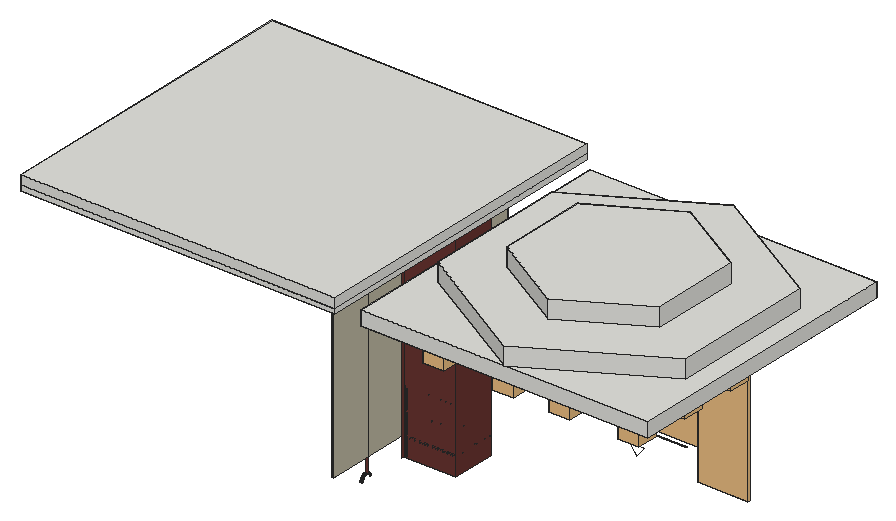
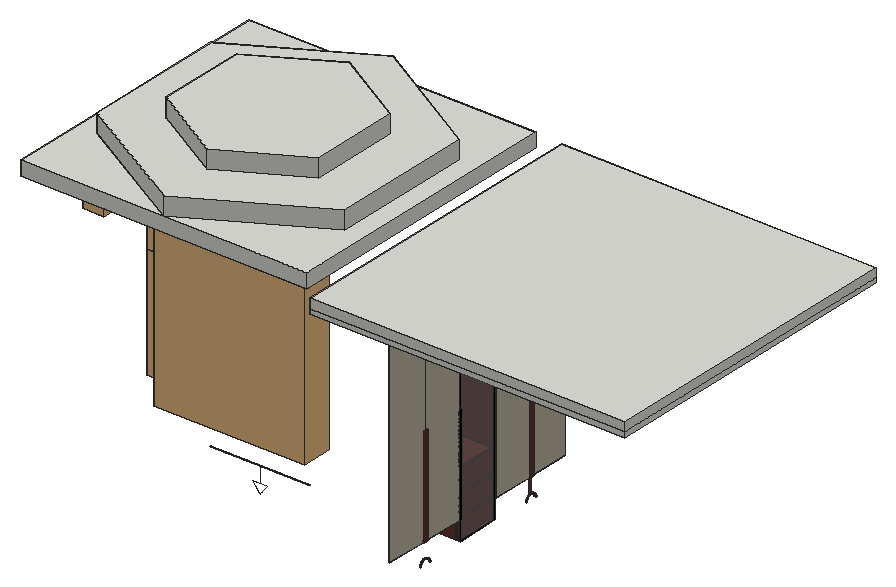
# SketchUp Ruby script. Lengths in millimetres.
U = 1.mm
M = Sketchup.active_model
def pt(a) = Geom::Point3d.new(a.map { |v| v * U })
def face(e, loops, mat)
  f = e.add_face(loops[0].map { |a| pt(a) })
  loops[1..].each { |l| e.add_face(l.map { |a| pt(a) }).erase! }
  f.material = f.back_material = mat if mat
  f
end
# faces: each face lists its corners as indices into pts; further lists are holes
def faces(e, pts, list, mat = nil) = list.each { |f| face(e, (f[0].is_a?(Array) ? f : [f]).map { |l| l.map { |i| pts[i] } }, mat) }
# xy, xz, yz: faces in a plane at the given z, y or x. An outline is a flat list of corners, or four numbers for a rectangle; further outlines are holes
def ring(l) = l.size == 4 ? [[l[0], l[1]], [l[2], l[1]], [l[2], l[3]], [l[0], l[3]]] : l.each_slice(2).to_a
def flat(e, list, mat, &to3) = list.each { |f| face(e, (f[0].is_a?(Array) ? f : [f]).map { |l| ring(l).map { |u, v| to3.(u, v) } }, mat) }
def xy(e, z, list, mat = nil) = flat(e, list, mat) { |x, y| [x, y, z] }
def xz(e, y, list, mat = nil) = flat(e, list, mat) { |x, z| [x, y, z] }
def yz(e, x, list, mat = nil) = flat(e, list, mat) { |y, z| [x, y, z] }
def lines(e, pts, list) = list.each { |a, b| e.add_line(pt(pts[a]), pt(pts[b])) }
# prism: a flat outline (further loops are holes) pulled along v
def prism(e, loops, v, mat = nil)
  f = face(e, loops, mat); d = Geom::Vector3d.new(v.map { |x| x * U })
  f.pushpull(f.normal.samedirection?(d) ? d.length : -d.length)
end
def box(e, o, s, mat = nil) = prism(e, [[o, [o[0] + s[0], o[1], o[2]], [o[0] + s[0], o[1] + s[1], o[2]], [o[0], o[1] + s[1], o[2]]]], [0, 0, s[2]], mat)
def at(x, y, z, deg = 0) = Geom::Transformation.translation(pt([x, y, z])) * Geom::Transformation.rotation(ORIGIN, Z_AXIS, deg.degrees)
def axes(o, x, y, z) = Geom::Transformation.new([*x, 0, *y, 0, *z, 0, *pt(o).to_a, 1])
def part(name) = M.definitions.add(name)
# library, detail: a bought-in or finely detailed component or shape, given as its bounding box
def library(name, o, s) = part(name).tap { |d| box(d.entities, o, s) }
def detail(e, o, s) = box(e.add_group.entities, o, s)
def put(e, d, t, mat = nil) = e.add_instance(d, t).tap { |i| i.material = mat if mat }
def group(e, t, mat = nil) = e.add_group.tap { |g| g.transformation = t; g.material = mat if mat }.entities
root = M.entities
M.materials.add("Olon-Fresh-Linen-VT10-1K").color = [226, 220, 209]
M.materials.add("Tafisa-Chateau-de-Sable-or-Sand-Castle-PM782-2K").color = [163, 138, 119]
M.materials.add("Uniboard-L17-Ambrette-4K").color = [104, 52, 49]
M.materials.add("Uniboard-L19-Putty-4K").color = [187, 181, 160]
M.materials.add("[Color M09]").color = [0, 0, 0]
M.materials.add("[Color M09]1").color = [0, 0, 0]
M.materials.add("[Translucent Glass Gray]").color = [128, 128, 128]
M.materials["[Translucent Glass Gray]"].alpha = 0.5
c1 = part("Group\#6")
prism(c1.entities,[[[0,248.3,178.4],[0,254.5,178.9],[0,259.6,180.5],[0,263.5,183.1],[0,266.3,186.7],[0,268,191.4],[0,268.6,197.1],[0,461,197.1],[0,461,0],[0,0,0],[0,0,197.1],[0,192.4,197.1],[0,193,191.4],[0,194.7,186.7],[0,197.5,183.1],[0,201.4,180.5],[0,206.5,178.9],[0,212.7,178.4]]],[18,0,0])
c2 = part("Group292\#1")
p = [[0,0,0],[0,0,-167.5],[-81.9,0,-167.5],[533.4,-9,0],[-533.4,-9,0],[533.4,9,0],
  [533.4,0,0],[-533.4,9,0],[81.9,0,-167.5],[-533.4,0,0],[0,0,-271.2]]
lines(c2.entities,p,[[0,1],[1,2],[3,4],[5,6],[7,5],[1,8],[9,0],[0,6],[8,10],[4,9],[6,3],[2,10],
  [9,7]])
c3 = part("Rectangle Light\#3")
put(c3.entities,c2,at(0,0,0))
c4 = part("Group\#4")
box(c4.entities,[12,0,-18],[547,461,18])
c5 = part("Group\#7")
prism(c5.entities,[[[20,25.4,1066.8],[20,17.4,1066.8],[20,12.1,1066.3],[20,7.7,1064.9],[20,4.3,1062.5],[20,1.9,1059.1],[20,0.5,1054.7],[20,0,1049.4],[20,0,17.4],[20,0.5,12.1],[20,1.9,7.7],[20,4.3,4.3],[20,7.7,1.9],[20,12.1,0.5],[20,17.4,0],[20,25.4,0]]],[-14,0,0])
c6 = library("Group\#29",[0,0,0],[533.4,18,1202.1])
c7 = library("Group\#23",[0,25.4,-404.8],[1600.2,330.2,1773.4])
c8 = library("Group\#28",[0,0,0],[533.4,18,709.7])
c9 = library("Group\#31",[0,0,0],[226.1,226.1,320.6])
c10 = part("Group\#17")
detail(c10.entities,[87.8,87.8,314.6],[50.5,50.5,6])
g1 = group(c10.entities,at(94.1,94.1,317.8))
xy(g1,0,[[17.2,0,12.4,1.1,8,3.4,4.3,6.8,1.7,11,0.2,15.7,0,20.7,1.1,25.6,3.4,30,6.8,33.6,11,36.3,15.7,37.8,20.7,37.9,25.6,36.8,30,34.5,33.6,31.2,36.3,27,37.8,22.2,37.9,17.2,36.8,12.4,34.5,8,31.2,4.3,27,1.7,22.2,0.2]])
box(root,[2628.9,2293.6,708.2],[18,454.2,2133.6],"Uniboard-L19-Putty-4K")
box(root,[2628.9,879.2,708.2],[18,454.2,2133.6],"Uniboard-L19-Putty-4K")
box(root,[2628.9,1336.4,708.2],[18,454.2,2133.6],"Uniboard-L19-Putty-4K")
xy(root,499.1,[[2628.9,1811.6,2646.9,2272.6]],"[Color M09]")
xy(root,546.1,[[2628.9,1332.9,2631.9,1333.4],[2631.9,1332.9,2646.9,1333.4]],"Tafisa-Chateau-de-Sable-or-Sand-Castle-PM782-2K")
xy(root,546.1,[[2619.9,1332.9,2628.9,1333.4],[2619.9,1336.4,2628.9,1336.9],[2616.9,2747.3,2628.9,2747.8],[2616.9,2750.8,2628.9,2751.3]],"Uniboard-L17-Ambrette-4K")
xy(root,705.2,[[2628.9,2293.6,2646.9,2747.8]],"Tafisa-Chateau-de-Sable-or-Sand-Castle-PM782-2K")
xy(root,705.2,[[2628.9,879.2,2646.9,1333.4],[2628.9,1336.4,2646.9,1790.6],[2628.9,2750.8,2646.9,3205]],"Uniboard-L17-Ambrette-4K")
xy(root,708.2,[[2628.9,2750.8,2646.9,3205]],"Uniboard-L19-Putty-4K")
xy(root,2823.8,[[2628.9,1811.6,2646.9,2272.6],[2649.9,1811.6,3208.9,2272.6]],"Uniboard-L17-Ambrette-4K")
xy(root,2841.8,[[2646.9,1793.6,2649.9,2290.6],[2628.9,2750.8,2646.9,3205]],"Uniboard-L19-Putty-4K")
xy(root,2841.8,[[2628.9,1793.6,2646.9,2290.6]],"[Color M09]")
xy(root,2844.8,[[2628.9,879.2,2646.9,3208]],"Uniboard-L19-Putty-4K")
xy(root,2895.6,[[2628.9,879.2,2646.9,3258.8],[2646.9,879.2,3238.5,3258.8]],"Uniboard-L19-Putty-4K")
xy(root,3048,[[5171.3,0,3851.4,762,3851.4,2286,5171.3,3048,6491.1,2286,6491.1,762]])
xy(root,3241.7,[[[5171.3,0,6491.1,762,6491.1,2286,5171.3,3048,3851.4,2286,3851.4,762],[5171.3,580.4,4354.1,1052.2,4354.1,1995.8,5171.3,2467.6,5988.4,1995.8,5988.4,1052.2]]])
xy(root,3435.4,[[5171.3,580.4,5988.4,1052.2,5988.4,1995.8,5171.3,2467.6,4354.1,1995.8,4354.1,1052.2]])
xz(root,879.2,[[2628.9,2844.8,2646.9,2895.6]],"Uniboard-L19-Putty-4K")
xz(root,1333.4,[[2628.9,546.1,2646.9,705.2]],"Uniboard-L17-Ambrette-4K")
xz(root,1811.6,[[2649.9,499.1,3208.9,2823.8]],"Uniboard-L17-Ambrette-4K")
xz(root,1811.6,[[2628.9,499.1,2646.9,2823.8]],"[Color M09]")
xz(root,2272.6,[[2649.9,499.1,3208.9,2823.8]],"Uniboard-L17-Ambrette-4K")
xz(root,2272.6,[[2628.9,499.1,2646.9,2823.8]],"[Color M09]")
xz(root,2750.8,[[2628.9,708.2,2646.9,2841.8]],"Uniboard-L19-Putty-4K")
xz(root,3205,[[2628.9,708.2,2646.9,2841.8]],"Uniboard-L19-Putty-4K")
yz(root,2628.9,[[2750.8,708.2,3205,2841.8]],"Uniboard-L19-Putty-4K")
yz(root,2637.9,[[1811.6,499.1,2272.6,2823.8]],"[Translucent Glass Gray]")
yz(root,2646.9,[[1793.6,499.1,1811.6,2823.8],[1793.6,2823.8,2290.6,2841.8]],"[Color M09]")
yz(root,2649.9,[[1793.6,499.1,1811.6,2823.8],[1793.6,2823.8,2290.6,2841.8]],"Uniboard-L17-Ambrette-4K")
yz(root,3208.9,[[1811.6,499.1,2272.6,2823.8]],"Uniboard-L17-Ambrette-4K")
yz(root,3851.4,[[762,3048,2286,3241.7]])
yz(root,4354.1,[[1052.2,3241.7,1995.8,3435.4]])
yz(root,5988.4,[[1052.2,3241.7,1995.8,3435.4]])
yz(root,6491.1,[[762,3048,2286,3241.7]])
p = [[2646.9,1270.2,487.2],[2631.9,1270.2,487.2],[2631.9,1270.4,489.2],[2646.9,1270.4,489.2],[2628.9,1270.4,489.2],[2628.9,1270.7,491.3],
  [2619.9,1270.7,491.3],[2619.9,1270.4,489.2],[2631.9,1270.7,491.3],[2646.9,1270.7,491.3],[2628.9,1399.1,491.3],[2628.9,1399.4,489.2],
  [2619.9,1399.4,489.2],[2619.9,1399.1,491.3],[2628.9,2684.8,489.2],[2628.9,2685.1,491.3],[2616.9,2685.1,491.3],[2616.9,2684.8,489.2],
  [2628.9,2813.5,491.3],[2628.9,2813.8,489.2],[2616.9,2813.8,489.2],[2616.9,2813.5,491.3],[2628.9,1271.1,493.3],[2619.9,1271.1,493.3],
  [2631.9,1271.1,493.3],[2646.9,1271.1,493.3],[2628.9,1398.8,493.3],[2619.9,1398.8,493.3],[2628.9,2685.5,493.3],[2616.9,2685.5,493.3],
  [2628.9,2813.2,493.3],[2616.9,2813.2,493.3],[2628.9,1271.5,495.3],[2619.9,1271.5,495.3],[2631.9,1271.5,495.3],[2646.9,1271.5,495.3],
  [2628.9,1398.3,495.3],[2619.9,1398.3,495.3],[2628.9,2685.9,495.3],[2616.9,2685.9,495.3],[2628.9,2812.7,495.3],[2616.9,2812.7,495.3],
  [2628.9,1271.9,497.3],[2619.9,1271.9,497.3],[2631.9,1271.9,497.3],[2646.9,1271.9,497.3],[2628.9,1397.9,497.3],[2619.9,1397.9,497.3],
  [2628.9,2686.3,497.3],[2616.9,2686.3,497.3],[2628.9,2812.3,497.3],[2616.9,2812.3,497.3],[2628.9,1272.5,499.2],[2619.9,1272.5,499.2],
  [2631.9,1272.5,499.2],[2646.9,1272.5,499.2],[2628.9,1397.3,499.2],[2619.9,1397.3,499.2],[2628.9,2686.9,499.2],[2616.9,2686.9,499.2],
  [2628.9,2811.7,499.2],[2616.9,2811.7,499.2],[2628.9,1273.1,501.2],[2619.9,1273.1,501.2],[2631.9,1273.1,501.2],[2646.9,1273.1,501.2],
  [2628.9,1396.7,501.2],[2619.9,1396.7,501.2],[2628.9,2687.5,501.2],[2616.9,2687.5,501.2],[2628.9,2811.1,501.2],[2616.9,2811.1,501.2],
  [2628.9,1273.7,503.1],[2619.9,1273.7,503.1],[2631.9,1273.7,503.1],[2646.9,1273.7,503.1],[2628.9,1396.1,503.1],[2619.9,1396.1,503.1],
  [2628.9,2688.1,503.1],[2616.9,2688.1,503.1],[2628.9,2810.5,503.1],[2616.9,2810.5,503.1],[2628.9,1274.5,505],[2619.9,1274.5,505],
  [2631.9,1274.5,505],[2646.9,1274.5,505],[2628.9,1395.3,505],[2619.9,1395.3,505],[2628.9,2688.9,505],[2616.9,2688.9,505],
  [2628.9,2809.7,505],[2616.9,2809.7,505],[2628.9,1275.3,506.9],[2619.9,1275.3,506.9],[2631.9,1275.3,506.9],[2646.9,1275.3,506.9],
  [2628.9,1394.6,506.9],[2619.9,1394.6,506.9],[2628.9,2689.7,506.9],[2616.9,2689.7,506.9],[2628.9,2809,506.9],[2616.9,2809,506.9],
  [2628.9,1276.1,508.8],[2619.9,1276.1,508.8],[2631.9,1276.1,508.8],[2646.9,1276.1,508.8],[2628.9,1393.7,508.8],[2619.9,1393.7,508.8],
  [2628.9,2690.5,508.8],[2616.9,2690.5,508.8],[2628.9,2808.1,508.8],[2616.9,2808.1,508.8],[2628.9,1277,510.6],[2619.9,1277,510.6],
  [2631.9,1277,510.6],[2646.9,1277,510.6],[2628.9,1392.8,510.6],[2619.9,1392.8,510.6],[2628.9,2691.4,510.6],[2616.9,2691.4,510.6],
  [2628.9,2807.2,510.6],[2616.9,2807.2,510.6],[2628.9,1277.9,512.4],[2619.9,1277.9,512.4],[2631.9,1277.9,512.4],[2646.9,1277.9,512.4],
  [2628.9,1391.9,512.4],[2619.9,1391.9,512.4],[2628.9,2692.3,512.4],[2616.9,2692.3,512.4],[2628.9,2806.3,512.4],[2616.9,2806.3,512.4],
  [2628.9,1279,514.2],[2619.9,1279,514.2],[2631.9,1279,514.2],[2646.9,1279,514.2],[2628.9,1390.9,514.2],[2619.9,1390.9,514.2],
  [2628.9,2693.4,514.2],[2616.9,2693.4,514.2],[2628.9,2805.3,514.2],[2616.9,2805.3,514.2],[2628.9,1280,515.9],[2619.9,1280,515.9],
  [2631.9,1280,515.9],[2646.9,1280,515.9],[2628.9,1389.8,515.9],[2619.9,1389.8,515.9],[2628.9,2694.4,515.9],[2616.9,2694.4,515.9],
  [2628.9,2804.2,515.9],[2616.9,2804.2,515.9],[2628.9,1281.1,517.6],[2619.9,1281.1,517.6],[2631.9,1281.1,517.6],[2646.9,1281.1,517.6],
  [2628.9,1388.7,517.6],[2619.9,1388.7,517.6],[2628.9,2695.5,517.6],[2616.9,2695.5,517.6],[2628.9,2803.1,517.6],[2616.9,2803.1,517.6],
  [2628.9,1282.3,519.3],[2619.9,1282.3,519.3],[2631.9,1282.3,519.3],[2646.9,1282.3,519.3],[2628.9,1387.5,519.3],[2619.9,1387.5,519.3],
  [2628.9,2696.7,519.3],[2616.9,2696.7,519.3],[2628.9,2801.9,519.3],[2616.9,2801.9,519.3],[2628.9,1283.5,520.9],[2619.9,1283.5,520.9],
  [2631.9,1283.5,520.9],[2646.9,1283.5,520.9],[2628.9,1386.3,520.9],[2619.9,1386.3,520.9],[2628.9,2697.9,520.9],[2616.9,2697.9,520.9],
  [2628.9,2800.7,520.9],[2616.9,2800.7,520.9],[2628.9,1284.8,522.5],[2619.9,1284.8,522.5],[2631.9,1284.8,522.5],[2646.9,1284.8,522.5],
  [2628.9,1385,522.5],[2619.9,1385,522.5],[2628.9,2699.2,522.5],[2616.9,2699.2,522.5],[2628.9,2799.4,522.5],[2616.9,2799.4,522.5],
  [2628.9,1286.1,524.1],[2619.9,1286.1,524.1],[2631.9,1286.1,524.1],[2646.9,1286.1,524.1],[2628.9,1383.7,524.1],[2619.9,1383.7,524.1],
  [2628.9,2700.5,524.1],[2616.9,2700.5,524.1],[2628.9,2798.1,524.1],[2616.9,2798.1,524.1],[2628.9,1287.5,525.6],[2619.9,1287.5,525.6],
  [2631.9,1287.5,525.6],[2646.9,1287.5,525.6],[2628.9,1382.3,525.6],[2619.9,1382.3,525.6],[2628.9,2701.9,525.6],[2616.9,2701.9,525.6],
  [2628.9,2796.7,525.6],[2616.9,2796.7,525.6],[2628.9,1288.9,527.1],[2619.9,1288.9,527.1],[2631.9,1288.9,527.1],[2646.9,1288.9,527.1],
  [2628.9,1380.9,527.1],[2619.9,1380.9,527.1],[2628.9,2703.3,527.1],[2616.9,2703.3,527.1],[2628.9,2795.3,527.1],[2616.9,2795.3,527.1],
  [2628.9,1290.4,528.5],[2619.9,1290.4,528.5],[2631.9,1290.4,528.5],[2646.9,1290.4,528.5],[2628.9,1379.4,528.5],[2619.9,1379.4,528.5],
  [2628.9,2704.8,528.5],[2616.9,2704.8,528.5],[2628.9,2793.8,528.5],[2616.9,2793.8,528.5],[2628.9,1291.9,529.9],[2619.9,1291.9,529.9],
  [2631.9,1291.9,529.9],[2646.9,1291.9,529.9],[2628.9,1377.9,529.9],[2619.9,1377.9,529.9],[2628.9,2706.3,529.9],[2616.9,2706.3,529.9],
  [2628.9,2792.3,529.9],[2616.9,2792.3,529.9],[2628.9,1293.5,531.2],[2619.9,1293.5,531.2],[2631.9,1293.5,531.2],[2646.9,1293.5,531.2],
  [2628.9,1376.3,531.2],[2619.9,1376.3,531.2],[2628.9,2707.9,531.2],[2616.9,2707.9,531.2],[2628.9,2790.7,531.2],[2616.9,2790.7,531.2],
  [2628.9,1295.1,532.5],[2619.9,1295.1,532.5],[2631.9,1295.1,532.5],[2646.9,1295.1,532.5],[2628.9,1374.7,532.5],[2619.9,1374.7,532.5],
  [2628.9,2709.5,532.5],[2616.9,2709.5,532.5],[2628.9,2789.1,532.5],[2616.9,2789.1,532.5],[2628.9,1296.7,533.7],[2619.9,1296.7,533.7],
  [2631.9,1296.7,533.7],[2646.9,1296.7,533.7],[2628.9,1373.1,533.7],[2619.9,1373.1,533.7],[2628.9,2711.1,533.7],[2616.9,2711.1,533.7],
  [2628.9,2787.5,533.7],[2616.9,2787.5,533.7],[2628.9,1298.4,534.9],[2619.9,1298.4,534.9],[2631.9,1298.4,534.9],[2646.9,1298.4,534.9],
  [2628.9,1371.4,534.9],[2619.9,1371.4,534.9],[2628.9,2712.8,534.9],[2616.9,2712.8,534.9],[2628.9,2785.8,534.9],[2616.9,2785.8,534.9],
  [2628.9,1300.1,536],[2619.9,1300.1,536],[2631.9,1300.1,536],[2646.9,1300.1,536],[2628.9,1369.7,536],[2619.9,1369.7,536],
  [2628.9,2714.5,536],[2616.9,2714.5,536],[2628.9,2784.1,536],[2616.9,2784.1,536],[2628.9,1301.8,537],[2619.9,1301.8,537],
  [2631.9,1301.8,537],[2646.9,1301.8,537],[2628.9,1368,537],[2619.9,1368,537],[2628.9,2716.2,537],[2616.9,2716.2,537],
  [2628.9,2782.4,537],[2616.9,2782.4,537],[2628.9,1303.6,538.1],[2619.9,1303.6,538.1],[2631.9,1303.6,538.1],[2646.9,1303.6,538.1],
  [2628.9,1366.2,538.1],[2619.9,1366.2,538.1],[2628.9,2718,538.1],[2616.9,2718,538.1],[2628.9,2780.6,538.1],[2616.9,2780.6,538.1],
  [2628.9,1305.4,539],[2619.9,1305.4,539],[2631.9,1305.4,539],[2646.9,1305.4,539],[2628.9,1364.4,539],[2619.9,1364.4,539],
  [2628.9,2719.8,539],[2616.9,2719.8,539],[2628.9,2778.8,539],[2616.9,2778.8,539],[2628.9,1307.2,539.9],[2619.9,1307.2,539.9],
  [2631.9,1307.2,539.9],[2646.9,1307.2,539.9],[2628.9,1362.6,539.9],[2619.9,1362.6,539.9],[2628.9,2721.6,539.9],[2616.9,2721.6,539.9],
  [2628.9,2777,539.9],[2616.9,2777,539.9],[2628.9,1309.1,540.8],[2619.9,1309.1,540.8],[2631.9,1309.1,540.8],[2646.9,1309.1,540.8],
  [2628.9,1360.7,540.8],[2619.9,1360.7,540.8],[2628.9,2723.5,540.8],[2616.9,2723.5,540.8],[2628.9,2775.1,540.8],[2616.9,2775.1,540.8],
  [2628.9,1311,541.5],[2619.9,1311,541.5],[2631.9,1311,541.5],[2646.9,1311,541.5],[2628.9,1358.8,541.5],[2619.9,1358.8,541.5],
  [2628.9,2725.4,541.5],[2616.9,2725.4,541.5],[2628.9,2773.2,541.5],[2616.9,2773.2,541.5],[2628.9,1312.9,542.3],[2619.9,1312.9,542.3],
  [2631.9,1312.9,542.3],[2646.9,1312.9,542.3],[2628.9,1356.9,542.3],[2619.9,1356.9,542.3],[2628.9,2727.3,542.3],[2616.9,2727.3,542.3],
  [2628.9,2771.3,542.3],[2616.9,2771.3,542.3],[2628.9,1314.8,542.9],[2619.9,1314.8,542.9],[2631.9,1314.8,542.9],[2646.9,1314.8,542.9],
  [2628.9,1355,542.9],[2619.9,1355,542.9],[2628.9,2729.2,542.9],[2616.9,2729.2,542.9],[2628.9,2769.4,542.9],[2616.9,2769.4,542.9],
  [2628.9,1316.8,543.5],[2619.9,1316.8,543.5],[2631.9,1316.8,543.5],[2646.9,1316.8,543.5],[2628.9,1353,543.5],[2619.9,1353,543.5],
  [2628.9,2731.2,543.5],[2616.9,2731.2,543.5],[2628.9,2767.4,543.5],[2616.9,2767.4,543.5],[2628.9,1318.7,544.1],[2619.9,1318.7,544.1],
  [2631.9,1318.7,544.1],[2646.9,1318.7,544.1],[2628.9,1351.1,544.1],[2619.9,1351.1,544.1],[2628.9,2733.1,544.1],[2616.9,2733.1,544.1],
  [2628.9,2765.5,544.1],[2616.9,2765.5,544.1],[2628.9,1320.7,544.5],[2619.9,1320.7,544.5],[2631.9,1320.7,544.5],[2646.9,1320.7,544.5],
  [2628.9,1349.1,544.5],[2619.9,1349.1,544.5],[2628.9,2735.1,544.5],[2616.9,2735.1,544.5],[2628.9,2763.5,544.5],[2616.9,2763.5,544.5],
  [2628.9,1322.7,544.9],[2619.9,1322.7,544.9],[2631.9,1322.7,544.9],[2646.9,1322.7,544.9],[2628.9,1347.1,544.9],[2619.9,1347.1,544.9],
  [2628.9,2737.1,544.9],[2616.9,2737.1,544.9],[2628.9,2761.5,544.9],[2616.9,2761.5,544.9],[2628.9,1324.7,545.3],[2619.9,1324.7,545.3],
  [2631.9,1324.7,545.3],[2646.9,1324.7,545.3],[2628.9,1345.1,545.3],[2619.9,1345.1,545.3],[2628.9,2739.1,545.3],[2616.9,2739.1,545.3],
  [2628.9,2759.5,545.3],[2616.9,2759.5,545.3],[2628.9,1326.8,545.6],[2619.9,1326.8,545.6],[2631.9,1326.8,545.6],[2646.9,1326.8,545.6],
  [2628.9,1343.1,545.6],[2619.9,1343.1,545.6],[2628.9,2741.2,545.6],[2616.9,2741.2,545.6],[2628.9,2757.5,545.6],[2616.9,2757.5,545.6],
  [2628.9,1328.8,545.8],[2619.9,1328.8,545.8],[2631.9,1328.8,545.8],[2646.9,1328.8,545.8],[2628.9,1341,545.8],[2619.9,1341,545.8],
  [2628.9,2743.2,545.8],[2616.9,2743.2,545.8],[2628.9,2755.4,545.8],[2616.9,2755.4,545.8],[2628.9,1330.8,546],[2619.9,1330.8,546],
  [2631.9,1330.8,546],[2646.9,1330.8,546],[2628.9,1339,546],[2619.9,1339,546],[2628.9,2745.2,546],[2616.9,2745.2,546],
  [2628.9,2753.4,546],[2616.9,2753.4,546],[2628.9,1332.9,546.1],[2619.9,1332.9,546.1],[2631.9,1332.9,546.1],[2646.9,1332.9,546.1],
  [2628.9,1336.9,546.1],[2619.9,1336.9,546.1],[2628.9,2747.3,546.1],[2616.9,2747.3,546.1],[2628.9,2751.3,546.1],[2616.9,2751.3,546.1],
  [3851.4,762,3048],[5171.3,0,3048],[5171.3,0,3241.7],[3851.4,762,3241.7],[6491.1,762,3048],[6491.1,762,3241.7],
  [5171.3,3048,3048],[3851.4,2286,3048],[3851.4,2286,3241.7],[5171.3,3048,3241.7],[6491.1,2286,3048],[6491.1,2286,3241.7],
  [4354.1,1052.2,3241.7],[5171.3,580.4,3241.7],[5171.3,580.4,3435.4],[4354.1,1052.2,3435.4],[5988.4,1052.2,3241.7],[5988.4,1052.2,3435.4],
  [5171.3,2467.6,3241.7],[4354.1,1995.8,3241.7],[4354.1,1995.8,3435.4],[5171.3,2467.6,3435.4],[5988.4,1995.8,3241.7],[5988.4,1995.8,3435.4],
  [2628.9,2749.3,546.1],[2628.9,2747.8,546.1],[2628.9,2750.8,546.1]]
faces(root,p,[[0,1,2,3],[5,8,2,4],[3,2,8,9],[22,24,8,5],[9,8,24,25],[32,34,24,22],[25,24,34,35],[42,44,34,32],
  [35,34,44,45],[52,54,44,42],[45,44,54,55],[62,64,54,52],[55,54,64,65],[72,74,64,62],[65,64,74,75],[82,84,74,72],
  [75,74,84,85],[92,94,84,82],[85,84,94,95],[102,104,94,92],[95,94,104,105],[112,114,104,102],[105,104,114,115],[122,124,114,112],
  [115,114,124,125],[132,134,124,122],[125,124,134,135],[142,144,134,132],[135,134,144,145],[152,154,144,142],[145,144,154,155],[162,164,154,152],
  [155,154,164,165],[172,174,164,162],[165,164,174,175],[182,184,174,172],[175,174,184,185],[192,194,184,182],[185,184,194,195],[202,204,194,192],
  [195,194,204,205],[212,214,204,202],[205,204,214,215],[222,224,214,212],[215,214,224,225],[232,234,224,222],[225,224,234,235],[242,244,234,232],
  [235,234,244,245],[252,254,244,242],[245,244,254,255],[262,264,254,252],[255,254,264,265],[272,274,264,262],[265,264,274,275],[282,284,274,272],
  [275,274,284,285],[292,294,284,282],[285,284,294,295],[302,304,294,292],[295,294,304,305],[312,314,304,302],[305,304,314,315],[322,324,314,312],
  [315,314,324,325],[332,334,324,322],[325,324,334,335],[342,344,334,332],[335,334,344,345],[352,354,344,342],[345,344,354,355],[362,364,354,352],
  [355,354,364,365],[372,374,364,362],[365,364,374,375],[382,384,374,372],[375,374,384,385],[392,394,384,382],[385,384,394,395],[402,404,394,392],
  [395,394,404,405],[412,414,404,402],[405,404,414,415],[422,424,414,412],[415,414,424,425],[432,434,424,422],[425,424,434,435],[442,444,434,432],
  [435,434,444,445],[452,454,444,442],[445,444,454,455]],"Tafisa-Chateau-de-Sable-or-Sand-Castle-PM782-2K")
faces(root,p,[[4,5,6,7],[10,11,12,13],[14,15,16,17],[18,19,20,21],[5,22,23,6],[26,10,13,27],[15,28,29,16],[30,18,21,31],
  [22,32,33,23],[36,26,27,37],[28,38,39,29],[40,30,31,41],[32,42,43,33],[46,36,37,47],[38,48,49,39],[50,40,41,51],
  [42,52,53,43],[56,46,47,57],[48,58,59,49],[60,50,51,61],[52,62,63,53],[66,56,57,67],[58,68,69,59],[70,60,61,71],
  [62,72,73,63],[76,66,67,77],[68,78,79,69],[80,70,71,81],[72,82,83,73],[86,76,77,87],[78,88,89,79],[90,80,81,91],
  [82,92,93,83],[96,86,87,97],[88,98,99,89],[100,90,91,101],[92,102,103,93],[106,96,97,107],[98,108,109,99],[110,100,101,111],
  [102,112,113,103],[116,106,107,117],[108,118,119,109],[120,110,111,121],[112,122,123,113],[126,116,117,127],[118,128,129,119],[130,120,121,131],
  [122,132,133,123],[136,126,127,137],[128,138,139,129],[140,130,131,141],[132,142,143,133],[146,136,137,147],[138,148,149,139],[150,140,141,151],
  [142,152,153,143],[156,146,147,157],[148,158,159,149],[160,150,151,161],[152,162,163,153],[166,156,157,167],[158,168,169,159],[170,160,161,171],
  [162,172,173,163],[176,166,167,177],[168,178,179,169],[180,170,171,181],[172,182,183,173],[186,176,177,187],[178,188,189,179],[190,180,181,191],
  [182,192,193,183],[196,186,187,197],[188,198,199,189],[200,190,191,201],[192,202,203,193],[206,196,197,207],[198,208,209,199],[210,200,201,211],
  [202,212,213,203],[216,206,207,217],[208,218,219,209],[220,210,211,221],[212,222,223,213],[226,216,217,227],[218,228,229,219],[230,220,221,231],
  [222,232,233,223],[236,226,227,237],[228,238,239,229],[240,230,231,241],[232,242,243,233],[246,236,237,247],[238,248,249,239],[250,240,241,251],
  [242,252,253,243],[256,246,247,257],[248,258,259,249],[260,250,251,261],[252,262,263,253],[266,256,257,267],[258,268,269,259],[270,260,261,271],
  [262,272,273,263],[276,266,267,277],[268,278,279,269],[280,270,271,281],[272,282,283,273],[286,276,277,287],[278,288,289,279],[290,280,281,291],
  [282,292,293,283],[296,286,287,297],[288,298,299,289],[300,290,291,301],[292,302,303,293],[306,296,297,307],[298,308,309,299],[310,300,301,311],
  [302,312,313,303],[316,306,307,317],[308,318,319,309],[320,310,311,321],[312,322,323,313],[326,316,317,327],[318,328,329,319],[330,320,321,331],
  [322,332,333,323],[336,326,327,337],[328,338,339,329],[340,330,331,341],[332,342,343,333],[346,336,337,347],[338,348,349,339],[350,340,341,351],
  [342,352,353,343],[356,346,347,357],[348,358,359,349],[360,350,351,361],[352,362,363,353],[366,356,357,367],[358,368,369,359],[370,360,361,371],
  [362,372,373,363],[376,366,367,377],[368,378,379,369],[380,370,371,381],[372,382,383,373],[386,376,377,387],[378,388,389,379],[390,380,381,391],
  [382,392,393,383],[396,386,387,397],[388,398,399,389],[400,390,391,401],[392,402,403,393],[406,396,397,407],[398,408,409,399],[410,400,401,411],
  [402,412,413,403],[416,406,407,417],[408,418,419,409],[420,410,411,421],[412,422,423,413],[426,416,417,427],[418,428,429,419],[430,420,421,431],
  [422,432,433,423],[436,426,427,437],[428,438,439,429],[440,430,431,441],[432,442,443,433],[446,436,437,447],[438,448,449,439],[450,440,441,451],
  [442,452,453,443],[456,446,447,457],[448,458,459,449],[460,450,451,461]],"Uniboard-L17-Ambrette-4K")
faces(root,p,[[462,463,464,465],[463,466,467,464],[468,469,470,471],[472,468,471,473],[474,475,476,477],[475,478,479,476],[480,481,482,483],[484,480,483,485]])
lines(root,p,[[486,487],[488,486]])
g2 = group(root,at(2649.9,1811.6,499.1),"Uniboard-L17-Ambrette-4K")
xy(g2,0,[[0,0,559,461]])
put(root,c1,axes([2661.9,1811.6,505.8],[1,0,0],[0,1,0],[0,0,0.96609]),"Uniboard-L17-Ambrette-4K")
put(root,c3,axes([4295,2858.6,894.1],[1,0,0],[0,-1,0],[0,0,1]))
put(root,c4,at(2649.9,1811.6,714.2),"Uniboard-L17-Ambrette-4K")
put(root,c5,at(2608.9,1308,708.2),"Uniboard-L17-Ambrette-4K")
put(root,c5,axes([2608.9,1361.8,708.2],[1,0,0],[0,-1,0],[0,0,1]),"Uniboard-L17-Ambrette-4K")
put(root,c5,at(2608.9,2722.4,708.2),"Uniboard-L17-Ambrette-4K")
put(root,c5,axes([2608.9,2776.2,708.2],[1,0,0],[0,-1,0],[0,0,1]),"Uniboard-L17-Ambrette-4K")
put(root,c5,at(2608.9,2265.2,708.2),"[Color M09]1")
put(root,c1,axes([2661.9,1811.6,717.2],[1,0,0],[0,1,0],[0,0,1.08549]),"Uniboard-L17-Ambrette-4K")
put(root,c4,at(2649.9,1811.6,949.1),"Uniboard-L17-Ambrette-4K")
put(root,c1,axes([2661.9,1811.6,952.1],[1,0,0],[0,1,0],[0,0,1.08549]),"Uniboard-L17-Ambrette-4K")
put(root,c6,at(5361.8,2342.1,977.8),"Olon-Fresh-Linen-VT10-1K")
put(root,c7,at(3761.6,2578.1,1524),"Olon-Fresh-Linen-VT10-1K")
put(root,c4,at(2649.9,1811.6,1184.1),"Uniboard-L17-Ambrette-4K")
put(root,c8,at(5361.8,2342.1,2182.9),"Olon-Fresh-Linen-VT10-1K")
put(root,c9,at(6089.4,2462.9,2565.1))
put(root,c9,at(5540,1875.3,2565.1))
put(root,c9,at(4078.6,2109.5,2572))
put(root,c9,at(4816.8,2109.5,2572))
put(root,c9,at(4078.6,1499.9,2572))
put(root,c9,at(4816.8,1499.9,2572))
put(root,c9,at(4078.6,890.3,2572))
put(root,c9,at(4816.8,890.3,2572))
put(root,c9,at(4078.6,280.7,2572))
put(root,c9,at(4816.8,280.7,2572))
put(root,c9,at(5416.9,1499.9,2572))
put(root,c9,at(6155.1,1499.9,2572))
put(root,c9,at(5416.9,280.7,2572))
put(root,c9,at(5416.9,890.3,2572))
put(root,c9,at(6155.1,280.7,2572))
put(root,c9,at(6155.1,890.3,2572))
put(root,c10,at(2203.5,2634.6,2575))
put(root,c10,at(2203.5,1245.5,2575))
put(root,c10,at(2203.5,1940.8,2575))
put(root,c10,at(2725.8,429.5,2575))
put(root,c10,at(1824.2,343.8,2575))
put(root,c10,at(570,343.8,2575))
put(root,c10,at(1197.1,343.8,2575))
put(root,c10,at(1208.6,2860.3,2575))
put(root,c10,at(267.2,2860.3,2575))
put(root,c10,at(178.3,1574.5,2575))
put(root,c10,at(178.3,688.6,2575))
put(root,c10,at(178.3,2484.1,2575))
g3 = group(root,at(0,20.3,2895.6))
xy(g3,0,[[[0,0,3352.8,3352.8],[631.1,520.7,1997.8,520.7,2066.4,526.9,2122.6,545.7,2166.3,576.9,2197.5,620.6,2216.3,676.8,2222.5,745.4,2222.5,2619.4,2216.3,2688,2197.5,2744.2,2166.3,2787.9,2122.6,2819.1,2066.4,2837.9,1997.8,2844.1,631.1,2844.1,562.5,2837.9,506.3,2819.1,462.6,2787.9,431.4,2744.2,412.6,2688,406.4,2619.4,406.4,745.4,412.6,676.8,431.4,620.6,462.6,576.9,506.3,545.7,562.5,526.9]]])
xy(g3,50.8,[[[0,0,3352.8,3352.8],[381,495.3,2298.7,2869.5]],[381,495.3,2222.5,520.7],[2222.5,495.3,2298.7,2844.1],[381,520.7,406.4,2844.1],[406.4,520.7,631.1,520.7,562.5,526.9,506.3,545.7,462.6,576.9,431.4,620.6,412.6,676.8,406.4,745.4],
  [1997.8,520.7,2222.5,520.7,2222.5,745.4,2216.3,676.8,2197.5,620.6,2166.3,576.9,2122.6,545.7,2066.4,526.9],[406.4,2619.4,412.6,2688,431.4,2744.2,462.6,2787.9,506.3,2819.1,562.5,2837.9,631.1,2844.1,406.4,2844.1],[2222.5,2619.4,2222.5,2844.1,1997.8,2844.1,2066.4,2837.9,2122.6,2819.1,2166.3,2787.9,2197.5,2744.2,2216.3,2688],[381,2844.1,2298.7,2869.5]])
xy(g3,101.6,[[381,495.3,2298.7,2869.5]])
xy(g3,152.4,[[0,0,3352.8,3352.8]])
xz(g3,0,[[0,0,3352.8,50.8],[0,50.8,3352.8,152.4]])
xz(g3,520.7,[[631.1,0,1997.8,50.8]])
xz(g3,2844.1,[[631.1,0,1997.8,50.8]])
xz(g3,3352.8,[[0,0,3352.8,50.8],[0,50.8,3352.8,152.4]])
yz(g3,0,[[0,0,3352.8,50.8],[0,50.8,3352.8,152.4]])
yz(g3,406.4,[[745.4,0,2619.4,50.8]])
yz(g3,2222.5,[[745.4,0,2619.4,50.8]])
yz(g3,3352.8,[[0,0,3352.8,50.8],[0,50.8,3352.8,152.4]])
p = [[631.1,520.7,50.8],[631.1,520.7,0],[562.5,526.9,0],[562.5,526.9,50.8],[1997.8,520.7,0],[1997.8,520.7,50.8],
  [2066.4,526.9,50.8],[2066.4,526.9,0],[506.3,545.7,0],[506.3,545.7,50.8],[2122.6,545.7,50.8],[2122.6,545.7,0],
  [462.6,576.9,0],[462.6,576.9,50.8],[2166.3,576.9,50.8],[2166.3,576.9,0],[431.4,620.6,0],[431.4,620.6,50.8],
  [2197.5,620.6,50.8],[2197.5,620.6,0],[412.6,676.8,0],[412.6,676.8,50.8],[2216.3,676.8,50.8],[2216.3,676.8,0],
  [406.4,745.4,0],[406.4,745.4,50.8],[2222.5,745.4,50.8],[2222.5,745.4,0],[406.4,2619.4,50.8],[406.4,2619.4,0],
  [412.6,2688,0],[412.6,2688,50.8],[2216.3,2688,50.8],[2216.3,2688,0],[2222.5,2619.4,0],[2222.5,2619.4,50.8],
  [431.4,2744.2,0],[431.4,2744.2,50.8],[2197.5,2744.2,50.8],[2197.5,2744.2,0],[462.6,2787.9,0],[462.6,2787.9,50.8],
  [2166.3,2787.9,50.8],[2166.3,2787.9,0],[506.3,2819.1,0],[506.3,2819.1,50.8],[2122.6,2819.1,50.8],[2122.6,2819.1,0],
  [562.5,2837.9,0],[562.5,2837.9,50.8],[2066.4,2837.9,50.8],[2066.4,2837.9,0],[631.1,2844.1,0],[631.1,2844.1,50.8],
  [1997.8,2844.1,50.8],[1997.8,2844.1,0]]
faces(g3,p,[[0,1,2,3],[4,5,6,7],[3,2,8,9],[7,6,10,11],[9,8,12,13],[11,10,14,15],[13,12,16,17],[15,14,18,19],
  [17,16,20,21],[19,18,22,23],[21,20,24,25],[23,22,26,27],[28,29,30,31],[32,33,34,35],[31,30,36,37],[38,39,33,32],
  [37,36,40,41],[42,43,39,38],[41,40,44,45],[46,47,43,42],[45,44,48,49],[50,51,47,46],[49,48,52,53],[54,55,51,50]])
g4 = group(g3,at(2298.7,495.3,50.8))
yz(g4,0,[[0,0,2374.2,50.8]])
g5 = group(g3,at(381,2869.5,50.8))
xz(g5,0,[[0,0,1917.7,50.8]])
g6 = group(g3,at(381,495.3,50.8))
xz(g6,0,[[0,0,1917.7,50.8]])
g7 = group(g3,at(381,495.3,50.8))
yz(g7,0,[[0,0,2374.2,50.8]])
g8 = group(root,at(3647.3,0,2895.6))
box(g8,[0,0,0],[3048,3048,152.4])
